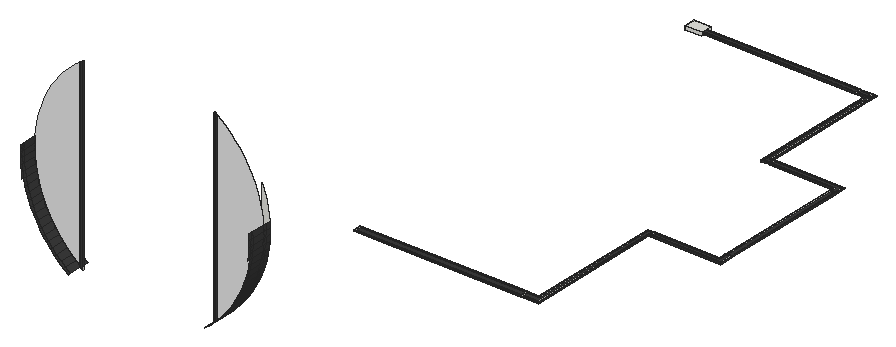
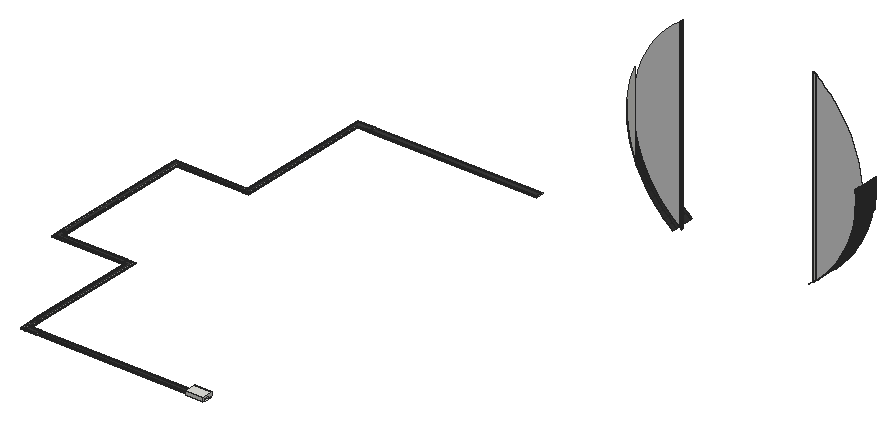
# SketchUp Ruby script. Lengths in inches.
U = 1.inch
M = Sketchup.active_model
def pt(a) = Geom::Point3d.new(a.map { |v| v * U })
def face(e, loops, mat)
  f = e.add_face(loops[0].map { |a| pt(a) })
  loops[1..].each { |l| e.add_face(l.map { |a| pt(a) }).erase! }
  f.material = f.back_material = mat if mat
  f
end
# faces: each face lists its corners as indices into pts; further lists are holes
def faces(e, pts, list, mat = nil) = list.each { |f| face(e, (f[0].is_a?(Array) ? f : [f]).map { |l| l.map { |i| pts[i] } }, mat) }
# xy, xz, yz: faces in a plane at the given z, y or x. An outline is a flat list of corners, or four numbers for a rectangle; further outlines are holes
def ring(l) = l.size == 4 ? [[l[0], l[1]], [l[2], l[1]], [l[2], l[3]], [l[0], l[3]]] : l.each_slice(2).to_a
def flat(e, list, mat, &to3) = list.each { |f| face(e, (f[0].is_a?(Array) ? f : [f]).map { |l| ring(l).map { |u, v| to3.(u, v) } }, mat) }
def xy(e, z, list, mat = nil) = flat(e, list, mat) { |x, y| [x, y, z] }
def xz(e, y, list, mat = nil) = flat(e, list, mat) { |x, z| [x, y, z] }
def yz(e, x, list, mat = nil) = flat(e, list, mat) { |y, z| [x, y, z] }
def lines(e, pts, list) = list.each { |a, b| e.add_line(pt(pts[a]), pt(pts[b])) }
# prism: a flat outline (further loops are holes) pulled along v
def prism(e, loops, v, mat = nil)
  f = face(e, loops, mat); d = Geom::Vector3d.new(v.map { |x| x * U })
  f.pushpull(f.normal.samedirection?(d) ? d.length : -d.length)
end
def box(e, o, s, mat = nil) = prism(e, [[o, [o[0] + s[0], o[1], o[2]], [o[0] + s[0], o[1] + s[1], o[2]], [o[0], o[1] + s[1], o[2]]]], [0, 0, s[2]], mat)
def at(x, y, z, deg = 0) = Geom::Transformation.translation(pt([x, y, z])) * Geom::Transformation.rotation(ORIGIN, Z_AXIS, deg.degrees)
def axes(o, x, y, z) = Geom::Transformation.new([*x, 0, *y, 0, *z, 0, *pt(o).to_a, 1])
def part(name) = M.definitions.add(name)
# library, detail: a bought-in or finely detailed component or shape, given as its bounding box
def library(name, o, s) = part(name).tap { |d| box(d.entities, o, s) }
def detail(e, o, s) = box(e.add_group.entities, o, s)
def put(e, d, t, mat = nil) = e.add_instance(d, t).tap { |i| i.material = mat if mat }
def group(e, t, mat = nil) = e.add_group.tap { |g| g.transformation = t; g.material = mat if mat }.entities
root = M.entities
M.materials.add("[Color M07]").color = [58, 58, 58]
M.materials.add("[Mirror 02]").color = [229, 229, 229]
xy(root,158,[[248.29,83.83,249,84.55],[165.63,84.55,248.29,87.25],[248.29,84.55,249,87.25],[249,84.55,249,87.25,255,87.25,255,155.13,257.29,155.13,257.29,153.49,256.57,153.49,256.57,84.55],[257.29,153.49,258,155.13],
  [258,153.49,258,155.13,290.75,155.13,290.75,159.3,292.7,159.3,292.7,153.49],[290.75,159.3,292.7,160.01],[290.75,160.01,292.7,224.11],[290.75,224.11,292.7,224.82],[290.75,224.82,290.75,227.13,258.71,227.13,258.71,229.11,292.7,229.11,292.7,224.82],
  [255,227.13,255,285.42,256.57,285.42,256.57,229.11,258,229.11,258,227.13],[258,227.13,258.71,229.11],[255,285.42,256.57,286.13],[255,286.13,255,291.4,255.73,291.4,255.73,293.99,256.57,293.99,256.57,286.13],[165.63,289.77,174.13,291.4],
  [164.9,291.4,165.63,294.72],[165.63,291.4,174.13,292.13],[255,291.4,255.5625,292.11],[255.5625,291.4,255.5625,292.11,255.02,292.11,255.02,292.13,255.5625,292.13,255.5625,293.99,255.73,293.99,255.73,291.4],[255,292.11,255.02,292.13],
  [165.63,292.13,249,293.99],[249,292.13,249.73,293.99],[249.73,292.13,255,293.99],[255,292.13,255.02,293.99],[255.02,292.13,255.5625,293.99],
  [165.63,293.99,174.13,294.72],[165.63,294.72,174.13,295.59]])
xy(root,158,[[164.92,83.83,164.92,87.97,248.29,87.97,248.29,87.25,165.63,87.25,165.63,84.55,248.29,84.55,248.29,83.83],[249,83.83,249,84.55,256.57,84.55,256.57,153.49,257.29,153.49,257.29,152.77,257.28,152.77,257.28,83.83],[248.29,87.25,249,87.97],[249,87.25,249,87.97,254.29,87.97,254.29,155.84,257.29,155.84,257.29,155.13,255,155.13,255,87.25],[257.29,152.77,258,153.49],
  [258,152.77,258,153.49,292.7,153.49,292.7,159.3,293.41,159.3,293.41,152.77],[257.29,155.13,258,155.84],[258,155.13,258,155.84,290.04,155.84,290.04,159.3,290.75,159.3,290.75,155.13],[290.04,159.3,290.75,160.01],[292.7,159.3,293.41,160.01],
  [290.04,160.01,290.75,224.11],[292.7,160.01,293.41,224.11],[290.04,224.11,290.75,224.82],[292.7,224.11,293.41,224.82],[290.04,224.82,290.04,226.42,258.71,226.42,258.71,227.13,290.75,227.13,290.75,224.82],
  [292.7,224.82,292.7,229.11,258.71,229.11,258.71,229.82,293.41,229.82,293.41,224.82],[254.29,226.42,254.29,285.42,255,285.42,255,227.13,258,227.13,258,226.42],[258,226.42,258.71,227.13],[256.57,229.11,256.57,285.42,257.28,285.42,257.28,229.82,258,229.82,258,229.11],[258,229.11,258.71,229.82],
  [254.29,285.42,255,286.13],[256.57,285.42,257.28,286.13],[254.29,286.13,255,291.4],[256.57,286.13,256.57,293.99,255.73,293.99,255.73,294.7,257.28,294.7,257.28,286.13],[174.13,291.4,249,292.13],
  [249,291.4,249.73,292.13],[249.73,291.4,249.73,292.13,255,292.13,255,292.11,254.29,292.11,254.29,291.4],[254.29,291.4,255,292.11],[174.13,293.99,249,294.72],[249,293.99,249.73,294.72],
  [249.73,293.99,249.73,294.72,255.73,294.72,255.73,294.7,255.02,294.7,255.02,293.99],[255.02,293.99,255.73,294.7]],"[Color M07]")
xy(root,158.5625,[[255,292.11,255.02,292.13]])
xy(root,158.5625,[[164.92,83.83,248.29,83.83,248.29,84.55,165.63,84.55,165.63,87.25,248.29,87.25,248.29,87.97,164.92,87.97],[248.29,83.83,249,84.55],[249,83.83,257.28,83.83,257.28,152.77,257.29,152.77,257.29,153.49,256.57,153.49,256.57,84.55,249,84.55],[165.63,84.55,248.29,87.25],[248.29,84.55,249,87.25],
  [249,84.55,256.57,84.55,256.57,153.49,257.29,153.49,257.29,155.13,255,155.13,255,87.25,249,87.25],[248.29,87.25,249,87.97],[249,87.25,255,87.25,255,155.13,257.29,155.13,257.29,155.84,254.29,155.84,254.29,87.97,249,87.97],[257.29,152.77,258,153.49],[258,152.77,293.41,152.77,293.41,159.3,292.7,159.3,292.7,153.49,258,153.49],
  [257.29,153.49,258,155.13],[258,153.49,292.7,153.49,292.7,159.3,290.75,159.3,290.75,155.13,258,155.13],[257.29,155.13,258,155.84],[258,155.13,290.75,155.13,290.75,159.3,290.04,159.3,290.04,155.84,258,155.84],[290.04,159.3,290.75,160.01],
  [290.75,159.3,292.7,160.01],[292.7,159.3,293.41,160.01],[290.04,160.01,290.75,224.11],[290.75,160.01,292.7,224.11],[292.7,160.01,293.41,224.11],
  [290.04,224.11,290.75,224.82],[290.75,224.11,292.7,224.82],[292.7,224.11,293.41,224.82],[290.04,224.82,290.75,224.82,290.75,227.13,258.71,227.13,258.71,226.42,290.04,226.42],[290.75,224.82,292.7,224.82,292.7,229.11,258.71,229.11,258.71,227.13,290.75,227.13],
  [292.7,224.82,293.41,224.82,293.41,229.82,258.71,229.82,258.71,229.11,292.7,229.11],[254.29,226.42,258,226.42,258,227.13,255,227.13,255,285.42,254.29,285.42],[258,226.42,258.71,227.13],[255,227.13,258,227.13,258,229.11,256.57,229.11,256.57,285.42,255,285.42],[258,227.13,258.71,229.11],
  [256.57,229.11,258,229.11,258,229.82,257.28,229.82,257.28,285.42,256.57,285.42],[258,229.11,258.71,229.82],[254.29,285.42,255,286.13],[255,285.42,256.57,286.13],[256.57,285.42,257.28,286.13],
  [254.29,286.13,255,291.4],[255,286.13,256.57,286.13,256.57,293.99,255.73,293.99,255.73,291.4,255,291.4],[256.57,286.13,257.28,286.13,257.28,294.7,255.73,294.7,255.73,293.99,256.57,293.99],[165.63,291.4,249,292.13],[249,291.4,249.73,292.13],
  [249.73,291.4,254.29,291.4,254.29,292.11,255,292.11,255,292.13,249.73,292.13],[254.29,291.4,255,292.11],[255,291.4,255.5625,292.11],[255.5625,291.4,255.73,291.4,255.73,293.99,255.5625,293.99,255.5625,292.13,255.02,292.13,255.02,292.11,255.5625,292.11],[165.63,292.13,249,293.99],
  [249,292.13,249.73,293.99],[249.73,292.13,255,293.99],[255,292.13,255.5625,293.99],[165.63,293.99,249,294.72],[249,293.99,249.73,294.72],
  [249.73,293.99,255.02,293.99,255.02,294.7,255.73,294.7,255.73,294.72,249.73,294.72],[255.02,293.99,255.73,294.7]],"[Color M07]")
xy(root,159.75,[[165.63,289.77,174.13,295.59]])
xz(root,32.53,[[70.64,129.99,70.64,223.45,69.46,222.61,69.46,130.82],[136.24,130.03,137.375,130.82,137.49,222.53,136.24,223.41]],"[Color M07]")
xz(root,33.16,[[70.64,129.99,69.46,130.82,69.46,222.61,70.64,223.45],[136.24,130.03,136.24,223.41,137.49,222.53,137.375,130.82]])
xz(root,33.16,[[69.46,130.82,69.46,222.61,69.34,222.53,66.95,220.65,64.66,218.65,62.48,216.52,60.42,214.29,58.48,211.94,56.67,209.5,54.99,206.96,53.45,204.34,52.05,201.64,50.79,198.87,49.6875,196.03,48.73,193.15,47.9375,190.21,47.3,187.24,46.82,184.23,46.5,181.21,46.34,178.17,46.34,175.125,46.51,172.09,46.84,169.0625,47.32,166.0625,47.97,163.09,48.78,160.15,49.74,157.27,50.85,154.4375,52.11,151.67,53.52,148.97,55.07,146.35,56.75,143.82,58.57,141.38,60.52,139.04,62.58,136.8125,64.77,134.69,67.06,132.69],[137.375,130.82,139.77,132.69,142.0625,134.69,144.25,136.8125,146.3125,139.04,148.26,141.38,150.08,143.82,151.76,146.35,153.3125,148.97,154.72,151.67,155.98,154.4375,157.09,157.27,158.05,160.15,158.86,163.09,159.51,166.0625,159.99,169.0625,160.32,172.09,160.49,175.125,160.49,178.17,160.33,181.21,160.01,184.23,159.53,187.24,158.89,190.21,158.09,193.15,157.14,196.03,156.04,198.87,154.78,201.64,153.38,204.34,151.84,206.96,150.16,209.5,148.35,211.94,146.41,214.29,144.35,216.52,142.17,218.65,139.88,220.65,137.49,222.53]],"[Mirror 02]")
xz(root,37.13,[[156.63,156.1,157.09,157.27,158.05,160.15,158.86,163.09,159.51,166.0625,159.99,169.0625,160.32,172.09,160.49,175.125,160.49,178.17,160.33,181.21,160.01,184.23,159.53,187.24,158.89,190.21,158.09,193.15,157.14,196.03,156.63,197.34]])
xz(root,83.83,[[164.92,158,248.29,158.5625],[248.29,158,249,158.5625],[249,158,257.28,158.5625]],"[Color M07]")
xz(root,84.55,[[165.63,158,248.29,158.5625],[248.29,158,249,158.5625],[249,158,256.57,158.5625]])
xz(root,87.25,[[165.63,158,248.29,158.5625],[248.29,158,249,158.5625],[249,158,255,158.5625]])
xz(root,87.97,[[164.92,158,248.29,158.5625],[248.29,158,249,158.5625],[249,158,254.29,158.5625]],"[Color M07]")
xz(root,152.77,[[257.28,158,257.29,158.5625]])
xz(root,152.77,[[257.29,158,258,158.5625],[258,158,293.41,158.5625]],"[Color M07]")
xz(root,153.49,[[256.57,158,257.29,158.5625],[257.29,158,258,158.5625],[258,158,292.7,158.5625]])
xz(root,155.13,[[255,158,257.29,158.5625],[257.29,158,258,158.5625],[258,158,290.75,158.5625]])
xz(root,155.84,[[254.29,158,257.29,158.5625],[257.29,158,258,158.5625],[258,158,290.04,158.5625]],"[Color M07]")
xz(root,159.3,[[290.04,158,290.75,158.5625],[290.75,158,292.7,158.5625],[292.7,158,293.41,158.5625]])
xz(root,160.01,[[290.04,158,290.75,158.5625],[290.75,158,292.7,158.5625],[292.7,158,293.41,158.5625]])
xz(root,224.11,[[290.04,158,290.75,158.5625],[290.75,158,292.7,158.5625],[292.7,158,293.41,158.5625]])
xz(root,224.82,[[290.04,158,290.75,158.5625],[290.75,158,292.7,158.5625],[292.7,158,293.41,158.5625]])
xz(root,226.42,[[254.29,158,258,158.5625],[258,158,258.71,158.5625],[258.71,158,290.04,158.5625]],"[Color M07]")
xz(root,227.13,[[255,158,258,158.5625],[258,158,258.71,158.5625],[258.71,158,290.75,158.5625]])
xz(root,229.11,[[256.57,158,258,158.5625],[258,158,258.71,158.5625],[258.71,158,292.7,158.5625]])
xz(root,229.82,[[257.28,158,258,158.5625],[258,158,258.71,158.5625],[258.71,158,293.41,158.5625]],"[Color M07]")
xz(root,285.42,[[254.29,158,255,158.5625],[255,158,256.57,158.5625],[256.57,158,257.28,158.5625]])
xz(root,286.13,[[254.29,158,255,158.5625],[255,158,256.57,158.5625],[256.57,158,257.28,158.5625]])
xz(root,289.77,[[165.63,158,174.13,159.75]])
xz(root,291.4,[[254.29,158,255,158.5625],[255,158,255.5625,158.5625],[255.5625,158,255.73,158.5625]])
xz(root,291.4,[[165.63,158,249,158.5625],[249,158,249.73,158.5625],[249.73,158,254.29,158.5625]],"[Color M07]")
xz(root,292.11,[[254.29,158,255,158.5625],[255,158,255.02,158.5625],[255.02,158,255.5625,158.5625]])
xz(root,292.13,[[165.63,158,249,158.5625],[249,158,249.73,158.5625],[249.73,158,255,158.5625],[255,158,255.02,158.5625],[255.02,158,255.5625,158.5625]])
xz(root,293.99,[[165.63,158,249,158.5625],[249,158,249.73,158.5625],[249.73,158,255,158.5625],[255,158,255.02,158.5625],[255.02,158,255.5625,158.5625],
  [255.5625,158,255.73,158.5625],[255.73,158,256.57,158.5625]])
xz(root,294.7,[[255.02,158,255.73,158.5625]])
xz(root,294.7,[[255.73,158,257.28,158.5625]],"[Color M07]")
xz(root,294.72,[[165.63,158,249,158.5625],[249,158,249.73,158.5625],[249.73,158,255.73,158.5625]],"[Color M07]")
xz(root,295.59,[[165.63,158,174.13,159.75]])
yz(root,46.34,[[24.2,175.125,25.27,178.17],[25.27,175.125,26.33,178.17],[26.33,175.125,33.16,178.17],[33.16,175.125,34.78,178.17],[34.78,175.125,37.13,178.17]],"[Color M07]")
yz(root,69.46,[[32.53,130.82,33.16,222.61]],"[Color M07]")
yz(root,70.64,[[32.53,129.99,33.16,131.66]])
yz(root,70.64,[[32.53,131.66,33.16,223.45]],"[Color M07]")
yz(root,136.24,[[32.53,130.03,33.16,223.41]],"[Color M07]")
yz(root,160.49,[[24.2,175.125,25.27,178.17],[25.27,175.125,26.33,178.17],[26.33,175.125,33.16,178.17],[33.16,175.125,34.78,178.17],[34.78,175.125,37.13,178.17]],"[Color M07]")
yz(root,164.92,[[83.83,158,87.97,158.5625]])
yz(root,165.63,[[84.55,158,87.25,158.5625],[289.77,158,291.4,158,291.4,158.5625,294.72,158.5625,294.72,158,295.59,158,295.59,159.75,289.77,159.75],[291.4,158,292.13,158.5625],[292.13,158,293.99,158.5625],[293.99,158,294.72,158.5625]])
yz(root,248.29,[[83.83,158,84.55,158.5625],[84.55,158,87.25,158.5625],[87.25,158,87.97,158.5625]])
yz(root,249,[[83.83,158,84.55,158.5625],[84.55,158,87.25,158.5625],[87.25,158,87.97,158.5625],[291.4,158,292.13,158.5625],[292.13,158,293.99,158.5625],
  [293.99,158,294.72,158.5625]])
yz(root,249.73,[[291.4,158,292.13,158.5625],[292.13,158,293.99,158.5625],[293.99,158,294.72,158.5625]])
yz(root,254.29,[[291.4,158,292.11,158.5625]])
yz(root,254.29,[[87.97,158,155.84,158.5625],[226.42,158,285.42,158.5625],[285.42,158,286.13,158.5625],[286.13,158,291.4,158.5625]],"[Color M07]")
yz(root,255,[[87.25,158,155.13,158.5625],[227.13,158,285.42,158.5625],[285.42,158,286.13,158.5625],[286.13,158,291.4,158.5625],[291.4,158,292.11,158.5625],
  [292.11,158,292.13,158.5625],[292.13,158,293.99,158.5625]])
yz(root,255.02,[[292.11,158,292.13,158.5625],[293.99,158,294.7,158.5625]])
yz(root,255.5625,[[291.4,158,292.11,158.5625],[292.13,158,293.99,158.5625]])
yz(root,255.73,[[291.4,158,293.99,158.5625],[293.99,158,294.7,158.5625]])
yz(root,255.73,[[294.7,158,294.72,158.5625]],"[Color M07]")
yz(root,256.57,[[84.55,158,153.49,158.5625],[229.11,158,285.42,158.5625],[285.42,158,286.13,158.5625],[286.13,158,293.99,158.5625]])
yz(root,257.28,[[83.83,158,152.77,158.5625],[229.82,158,285.42,158.5625],[285.42,158,286.13,158.5625],[286.13,158,294.7,158.5625]],"[Color M07]")
yz(root,257.29,[[152.77,158,153.49,158.5625],[153.49,158,155.13,158.5625],[155.13,158,155.84,158.5625]])
yz(root,258,[[152.77,158,153.49,158.5625],[153.49,158,155.13,158.5625],[155.13,158,155.84,158.5625],[226.42,158,227.13,158.5625],[227.13,158,229.11,158.5625],
  [229.11,158,229.82,158.5625]])
yz(root,258.71,[[226.42,158,227.13,158.5625],[227.13,158,229.11,158.5625],[229.11,158,229.82,158.5625]])
yz(root,290.04,[[155.84,158,159.3,158.5625],[159.3,158,160.01,158.5625],[160.01,158,224.11,158.5625],[224.11,158,224.82,158.5625],[224.82,158,226.42,158.5625]],"[Color M07]")
yz(root,290.75,[[155.13,158,159.3,158.5625],[159.3,158,160.01,158.5625],[160.01,158,224.11,158.5625],[224.11,158,224.82,158.5625],[224.82,158,227.13,158.5625]])
yz(root,292.7,[[153.49,158,159.3,158.5625],[159.3,158,160.01,158.5625],[160.01,158,224.11,158.5625],[224.11,158,224.82,158.5625],[224.82,158,229.11,158.5625]])
yz(root,293.41,[[152.77,158,159.3,158.5625],[159.3,158,160.01,158.5625],[160.01,158,224.11,158.5625],[224.11,158,224.82,158.5625],[224.82,158,229.82,158.5625]],"[Color M07]")
p = [[70.64,33.16,129.99],[69.46,33.16,130.82],[69.46,32.53,130.82],[70.64,32.53,129.99],[137.375,33.16,130.82],[136.24,33.16,130.03],
  [136.24,32.53,130.03],[137.375,32.53,130.82],[69.46,25.27,130.82],[69.46,26.33,130.82],[67.06,26.33,132.69],[67.06,25.27,132.69],
  [139.77,25.27,132.69],[139.77,26.33,132.69],[137.375,26.33,130.82],[137.375,25.27,130.82],[67.06,33.16,132.69],[139.77,33.16,132.69],
  [137.49,33.16,222.53],[137.49,32.53,222.53],[67.06,34.78,132.69],[69.46,34.78,130.82],[137.375,34.78,130.82],[139.77,34.78,132.69],
  [67.06,37.13,132.69],[69.46,37.13,130.82],[137.375,37.13,130.82],[139.77,37.13,132.69],[64.77,26.33,134.69],[64.77,25.27,134.69],
  [142.0625,25.27,134.69],[142.0625,26.33,134.69],[64.77,33.16,134.69],[142.0625,33.16,134.69],[64.77,34.78,134.69],[142.0625,34.78,134.69],
  [64.77,37.13,134.69],[142.0625,37.13,134.69],[62.58,26.33,136.8125],[62.58,25.27,136.8125],[144.25,25.27,136.8125],[144.25,26.33,136.8125],
  [62.58,33.16,136.8125],[144.25,33.16,136.8125],[62.58,34.78,136.8125],[144.25,34.78,136.8125],[62.58,37.13,136.8125],[144.25,37.13,136.8125],
  [60.52,26.33,139.04],[60.52,25.27,139.04],[146.3125,25.27,139.04],[146.3125,26.33,139.04],[60.52,33.16,139.04],[146.3125,33.16,139.04],
  [60.52,34.78,139.04],[146.3125,34.78,139.04],[60.52,37.13,139.04],[146.3125,37.13,139.04],[58.57,26.33,141.38],[58.57,25.27,141.38],
  [148.26,25.27,141.38],[148.26,26.33,141.38],[58.57,33.16,141.38],[148.26,33.16,141.38],[58.57,34.78,141.38],[148.26,34.78,141.38],
  [58.57,37.13,141.38],[148.26,37.13,141.38],[56.75,26.33,143.82],[56.75,25.27,143.82],[150.08,25.27,143.82],[150.08,26.33,143.82],
  [56.75,33.16,143.82],[150.08,33.16,143.82],[56.75,34.78,143.82],[150.08,34.78,143.82],[56.75,37.13,143.82],[150.08,37.13,143.82],
  [55.07,26.33,146.35],[55.07,25.27,146.35],[151.76,25.27,146.35],[151.76,26.33,146.35],[55.07,33.16,146.35],[151.76,33.16,146.35],
  [55.07,34.78,146.35],[151.76,34.78,146.35],[55.07,37.13,146.35],[151.76,37.13,146.35],[53.52,26.33,148.97],[53.52,25.27,148.97],
  [153.3125,25.27,148.97],[153.3125,26.33,148.97],[53.52,33.16,148.97],[153.3125,33.16,148.97],[53.52,34.78,148.97],[153.3125,34.78,148.97],
  [53.52,37.13,148.97],[153.3125,37.13,148.97],[52.11,26.33,151.67],[52.11,25.27,151.67],[154.72,25.27,151.67],[154.72,26.33,151.67],
  [52.11,33.16,151.67],[154.72,33.16,151.67],[52.11,34.78,151.67],[154.72,34.78,151.67],[52.11,37.13,151.67],[154.72,37.13,151.67],
  [50.85,26.33,154.4375],[50.85,25.27,154.4375],[155.98,25.27,154.4375],[155.98,26.33,154.4375],[50.85,33.16,154.4375],[155.98,33.16,154.4375],
  [50.85,34.78,154.4375],[155.98,34.78,154.4375],[50.85,37.13,154.4375],[155.98,37.13,154.4375],[49.74,26.33,157.27],[49.74,25.27,157.27],
  [157.09,25.27,157.27],[157.09,26.33,157.27],[49.74,33.16,157.27],[157.09,33.16,157.27],[49.74,34.78,157.27],[157.09,34.78,157.27],
  [49.74,37.13,157.27],[157.09,37.13,157.27],[156.63,37.13,156.1],[48.78,26.33,160.15],[48.78,25.27,160.15],[158.05,25.27,160.15],
  [158.05,26.33,160.15],[48.78,33.16,160.15],[158.05,33.16,160.15],[48.78,34.78,160.15],[158.05,34.78,160.15],[48.78,37.13,160.15],
  [158.05,37.13,160.15],[47.97,26.33,163.09],[47.97,25.27,163.09],[158.86,25.27,163.09],[158.86,26.33,163.09],[47.97,33.16,163.09],
  [158.86,33.16,163.09],[47.97,34.78,163.09],[158.86,34.78,163.09],[47.97,37.13,163.09],[158.86,37.13,163.09],[47.32,26.33,166.0625],
  [47.32,25.27,166.0625],[159.51,25.27,166.0625],[159.51,26.33,166.0625],[47.32,33.16,166.0625],[159.51,33.16,166.0625],[47.32,34.78,166.0625],
  [159.51,34.78,166.0625],[47.32,37.13,166.0625],[159.51,37.13,166.0625],[47.32,24.2,166.0625],[46.84,25.27,169.0625],[46.84,24.2,169.0625],
  [46.84,26.33,169.0625],[159.99,25.27,169.0625],[159.99,26.33,169.0625],[46.84,33.16,169.0625],[159.99,33.16,169.0625],[46.84,34.78,169.0625],
  [159.99,34.78,169.0625],[46.84,37.13,169.0625],[159.99,37.13,169.0625],[46.51,25.27,172.09],[46.51,24.2,172.09],[160.32,24.2,172.09],
  [160.32,25.27,172.09],[159.99,24.2,169.0625],[46.51,26.33,172.09],[160.32,26.33,172.09],[46.51,33.16,172.09],[160.32,33.16,172.09],
  [46.51,34.78,172.09],[160.32,34.78,172.09],[46.51,37.13,172.09],[160.32,37.13,172.09],[46.34,25.27,175.125],[46.34,24.2,175.125],
  [160.49,24.2,175.125],[160.49,25.27,175.125],[46.34,26.33,175.125],[160.49,26.33,175.125],[46.34,33.16,175.125],[160.49,33.16,175.125],
  [46.34,34.78,175.125],[160.49,34.78,175.125],[46.34,37.13,175.125],[160.49,37.13,175.125],[46.34,24.2,178.17],[46.34,25.27,178.17],
  [46.5,25.27,181.21],[46.5,24.2,181.21],[160.33,24.2,181.21],[160.33,25.27,181.21],[160.49,25.27,178.17],[160.49,24.2,178.17],
  [46.34,26.33,178.17],[46.5,26.33,181.21],[160.33,26.33,181.21],[160.49,26.33,178.17],[46.34,33.16,178.17],[46.5,33.16,181.21],
  [160.33,33.16,181.21],[160.49,33.16,178.17],[46.5,34.78,181.21],[46.34,34.78,178.17],[160.49,34.78,178.17],[160.33,34.78,181.21],
  [46.5,37.13,181.21],[46.34,37.13,178.17],[160.49,37.13,178.17],[160.33,37.13,181.21]]
faces(root,p,[[0,1,2,3],[4,5,6,7]])
faces(root,p,[[8,9,10,11],[12,13,14,15],[2,1,16,10,9],[13,17,4,7,14],[4,18,19,7],[20,21,1,16],[22,23,17,4],[24,20,21,25],
  [26,22,23,27],[11,10,28,29],[30,31,13,12],[10,16,32,28],[31,33,17,13],[34,20,16,32],[23,35,33,17],[36,34,20,24],
  [27,23,35,37],[29,28,38,39],[40,41,31,30],[28,32,42,38],[41,43,33,31],[44,34,32,42],[35,45,43,33],[46,44,34,36],
  [37,35,45,47],[39,38,48,49],[50,51,41,40],[38,42,52,48],[51,53,43,41],[54,44,42,52],[45,55,53,43],[56,54,44,46],
  [47,45,55,57],[49,48,58,59],[60,61,51,50],[48,52,62,58],[61,63,53,51],[64,54,52,62],[55,65,63,53],[66,64,54,56],
  [57,55,65,67],[59,58,68,69],[70,71,61,60],[58,62,72,68],[71,73,63,61],[74,64,62,72],[65,75,73,63],[76,74,64,66],
  [67,65,75,77],[69,68,78,79],[80,81,71,70],[68,72,82,78],[81,83,73,71],[84,74,72,82],[75,85,83,73],[86,84,74,76],
  [77,75,85,87],[79,78,88,89],[90,91,81,80],[78,82,92,88],[91,93,83,81],[94,84,82,92],[85,95,93,83],[96,94,84,86],
  [87,85,95,97],[89,88,98,99],[100,101,91,90],[88,92,102,98],[101,103,93,91],[104,94,92,102],[95,105,103,93],[106,104,94,96],
  [97,95,105,107],[99,98,108,109],[110,111,101,100],[98,102,112,108],[111,113,103,101],[114,104,102,112],[105,115,113,103],[116,114,104,106],
  [107,105,115,117],[109,108,118,119],[120,121,111,110],[108,112,122,118],[121,123,113,111],[124,114,112,122],[115,125,123,113],[126,124,114,116],
  [117,115,125,127,128],[119,118,129,130],[131,132,121,120],[118,122,133,129],[132,134,123,121],[135,124,122,133],[125,136,134,123],[137,135,124,126],
  [127,125,136,138],[130,129,139,140],[141,142,132,131],[129,133,143,139],[142,144,134,132],[145,135,133,143],[136,146,144,134],[147,145,135,137],
  [138,136,146,148],[140,139,149,150],[151,152,142,141],[139,143,153,149],[152,154,144,142],[155,145,143,153],[146,156,154,144],[157,155,145,147],
  [148,146,156,158],[159,150,160,161],[150,149,162,160],[163,164,152,151],[149,153,165,162],[164,166,154,152],[167,155,153,165],[156,168,166,154],
  [169,167,155,157],[158,156,168,170],[161,160,171,172],[173,174,163,175],[160,162,176,171],[174,177,164,163],[162,165,178,176],[177,179,166,164],
  [180,167,165,178],[168,181,179,166],[182,180,167,169],[170,168,181,183],[172,171,184,185],[186,187,174,173],[171,176,188,184],[187,189,177,174],
  [176,178,190,188],[189,191,179,177],[192,180,178,190],[181,193,191,179],[194,192,180,182],[183,181,193,195],[196,197,198,199],[200,201,202,203],
  [197,204,205,198],[201,206,207,202],[204,208,209,205],[206,210,211,207],[212,213,208,209],[214,215,210,211],[216,212,213,217],[218,214,215,219]],"[Color M07]")
